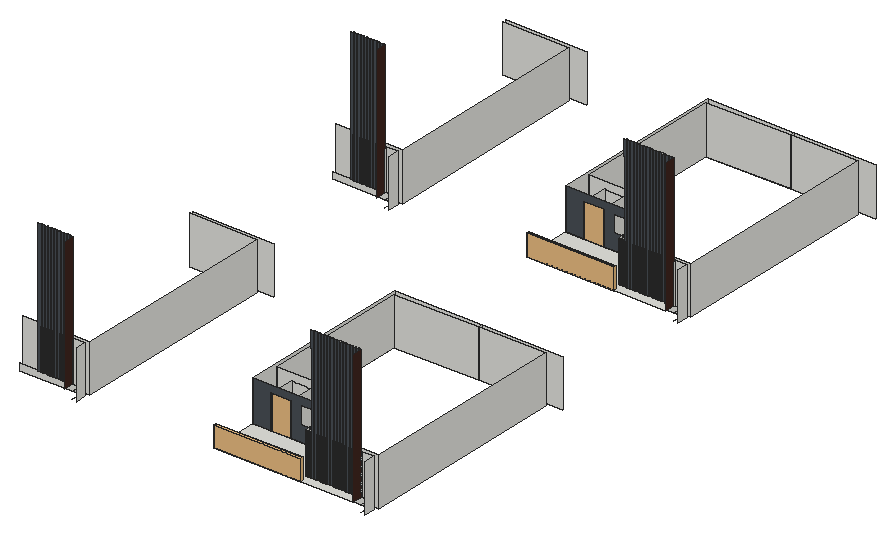
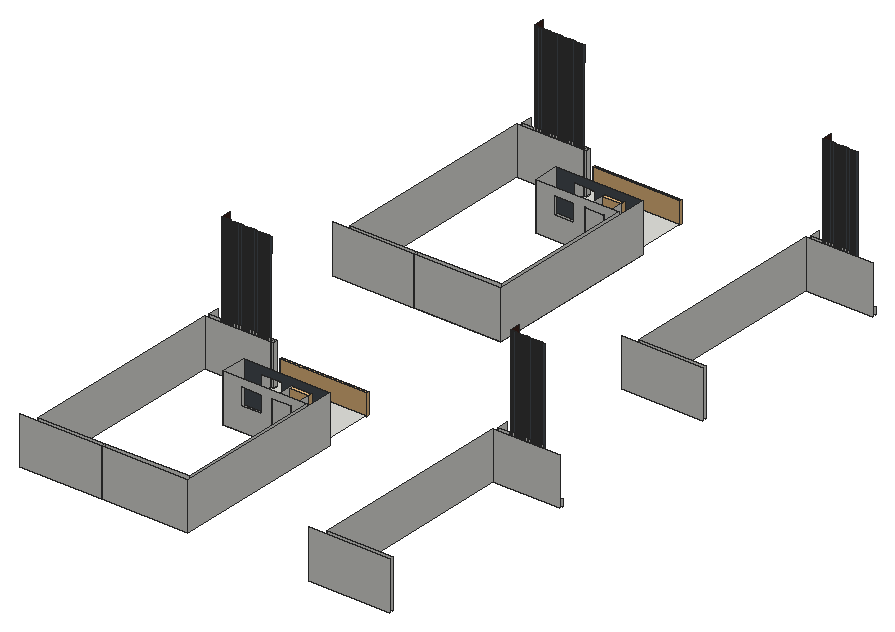
# SketchUp Ruby script. Lengths in inches.
U = 1.inch
M = Sketchup.active_model
def pt(a) = Geom::Point3d.new(a.map { |v| v * U })
def face(e, loops, mat)
  f = e.add_face(loops[0].map { |a| pt(a) })
  loops[1..].each { |l| e.add_face(l.map { |a| pt(a) }).erase! }
  f.material = f.back_material = mat if mat
  f
end
# faces: each face lists its corners as indices into pts; further lists are holes
def faces(e, pts, list, mat = nil) = list.each { |f| face(e, (f[0].is_a?(Array) ? f : [f]).map { |l| l.map { |i| pts[i] } }, mat) }
# xy, xz, yz: faces in a plane at the given z, y or x. An outline is a flat list of corners, or four numbers for a rectangle; further outlines are holes
def ring(l) = l.size == 4 ? [[l[0], l[1]], [l[2], l[1]], [l[2], l[3]], [l[0], l[3]]] : l.each_slice(2).to_a
def flat(e, list, mat, &to3) = list.each { |f| face(e, (f[0].is_a?(Array) ? f : [f]).map { |l| ring(l).map { |u, v| to3.(u, v) } }, mat) }
def xy(e, z, list, mat = nil) = flat(e, list, mat) { |x, y| [x, y, z] }
def xz(e, y, list, mat = nil) = flat(e, list, mat) { |x, z| [x, y, z] }
def yz(e, x, list, mat = nil) = flat(e, list, mat) { |y, z| [x, y, z] }
def lines(e, pts, list) = list.each { |a, b| e.add_line(pt(pts[a]), pt(pts[b])) }
# prism: a flat outline (further loops are holes) pulled along v
def prism(e, loops, v, mat = nil)
  f = face(e, loops, mat); d = Geom::Vector3d.new(v.map { |x| x * U })
  f.pushpull(f.normal.samedirection?(d) ? d.length : -d.length)
end
def box(e, o, s, mat = nil) = prism(e, [[o, [o[0] + s[0], o[1], o[2]], [o[0] + s[0], o[1] + s[1], o[2]], [o[0], o[1] + s[1], o[2]]]], [0, 0, s[2]], mat)
def at(x, y, z, deg = 0) = Geom::Transformation.translation(pt([x, y, z])) * Geom::Transformation.rotation(ORIGIN, Z_AXIS, deg.degrees)
def axes(o, x, y, z) = Geom::Transformation.new([*x, 0, *y, 0, *z, 0, *pt(o).to_a, 1])
def part(name) = M.definitions.add(name)
# library, detail: a bought-in or finely detailed component or shape, given as its bounding box
def library(name, o, s) = part(name).tap { |d| box(d.entities, o, s) }
def detail(e, o, s) = box(e.add_group.entities, o, s)
def put(e, d, t, mat = nil) = e.add_instance(d, t).tap { |i| i.material = mat if mat }
def group(e, t, mat = nil) = e.add_group.tap { |g| g.transformation = t; g.material = mat if mat }.entities
root = M.entities
M.materials.add("[0043_SaddleBrown]").color = [63, 38, 31]
M.materials.add("[Formica Blue]").color = [73, 80, 86]
c1 = library("door (1)",[38.93,25.48,0],[40,9.94,82.68])
c2 = library("Glass Railing",[0,0,0],[139.5,4.76,42])
xy(root,384.25,[[1797.0625,438.72,1802.84,447.84],[1586.375,535.375,1586.375,980.35,1802.84,980.35,1802.84,971.23,1593.72,965.96,1593.72,540.48,1802.84,540.48,1802.84,535.375],[1593.72,540.48,1802.84,598.8125],[1797.0625,1419.07,1802.84,1428.19],[1586.375,1515.73,1586.375,1960.7,1802.84,1960.7,1802.84,1951.58,1593.72,1946.3125,1593.72,1520.83,1802.84,1520.83,1802.84,1515.73],
  [1593.72,1520.83,1802.84,1579.16]])
xy(root,401.6875,[[1586.375,412.04,1935.9375,412.04,1935.9375,437.1,1930.18,437.1,1930.18,438.72,1927.9375,438.72,1927.9375,437.1,1922.18,437.1,1922.18,438.72,1919.9375,438.72,1919.9375,437.1,1914.18,437.1,1914.18,438.72,1911.9375,438.72,1911.9375,437.1,1906.18,437.1,1906.18,438.72,1903.9375,438.72,1903.9375,437.1,1898.18,437.1,1898.18,438.72,1895.9375,438.72,1895.9375,437.1,1890.18,437.1,1890.18,438.72,1887.9375,438.72,1887.9375,437.1,1882.18,437.1,1882.18,438.72,1879.9375,438.72,1879.9375,437.1,1874.18,437.1,1874.18,438.72,1871.9375,438.72,1871.9375,437.1,1866.18,437.1,1866.18,438.72,1863.9375,438.72,1863.9375,437.1,1858.18,437.1,1858.18,438.72,1855.9375,438.72,1855.9375,437.1,1850.18,437.1,1850.18,438.72,1847.9375,438.72,1847.9375,437.1,1842.18,437.1,1842.18,438.72,1839.9375,438.72,1839.9375,437.1,1834.18,437.1,1834.18,438.72,1831.9375,438.72,1831.9375,437.1,1826.18,437.1,1826.18,438.72,1823.9375,438.72,1823.9375,437.1,1818.18,437.1,1818.18,438.72,1815.9375,438.72,1815.9375,437.1,1810.18,437.1,1810.18,438.72,1807.75,438.72,1807.75,437.1,1802.84,437.1,1802.84,438.72,1801.29,438.72,1801.29,437.1,1797.0625,437.1,1797.0625,447.84,1802.84,447.84,1802.84,535.375,1586.375,535.375],[1133.74,437.1,1139.5,438.72],[1141.74,437.1,1147.5,438.72],[1149.74,437.1,1155.5,438.72],[1157.74,437.1,1163.5,438.72],
  [1165.74,437.1,1171.5,438.72],[1173.74,437.1,1179.5,438.72],[1181.74,437.1,1187.5,438.72],[1189.74,437.1,1195.5,438.72],[1197.74,437.1,1203.5,438.72],
  [1205.74,437.1,1211.5,438.72],[1797.0625,437.1,1801.29,438.72],[1802.84,437.1,1807.75,438.72],[1810.18,437.1,1815.9375,438.72],[1818.18,437.1,1823.9375,438.72],
  [1826.18,437.1,1831.9375,438.72],[1834.18,437.1,1839.9375,438.72],[1842.18,437.1,1847.9375,438.72],[1850.18,437.1,1855.9375,438.72],[1858.18,437.1,1863.9375,438.72],
  [1866.18,437.1,1871.9375,438.72],[1874.18,437.1,1879.9375,438.72],[1882.18,437.1,1887.9375,438.72],[1890.18,437.1,1895.9375,438.72],[1898.18,437.1,1903.9375,438.72],
  [1906.18,437.1,1911.9375,438.72],[1914.18,437.1,1919.9375,438.72],[1922.18,437.1,1927.9375,438.72],[1930.18,437.1,1935.9375,438.72],[1632.17,535.375,1680.17,598.8125],
  [1586.375,1392.39,1935.9375,1392.39,1935.9375,1417.45,1930.18,1417.45,1930.18,1419.07,1927.9375,1419.07,1927.9375,1417.45,1922.18,1417.45,1922.18,1419.07,1919.9375,1419.07,1919.9375,1417.45,1914.18,1417.45,1914.18,1419.07,1911.9375,1419.07,1911.9375,1417.45,1906.18,1417.45,1906.18,1419.07,1903.9375,1419.07,1903.9375,1417.45,1898.18,1417.45,1898.18,1419.07,1895.9375,1419.07,1895.9375,1417.45,1890.18,1417.45,1890.18,1419.07,1887.9375,1419.07,1887.9375,1417.45,1882.18,1417.45,1882.18,1419.07,1879.9375,1419.07,1879.9375,1417.45,1874.18,1417.45,1874.18,1419.07,1871.9375,1419.07,1871.9375,1417.45,1866.18,1417.45,1866.18,1419.07,1863.9375,1419.07,1863.9375,1417.45,1858.18,1417.45,1858.18,1419.07,1855.9375,1419.07,1855.9375,1417.45,1850.18,1417.45,1850.18,1419.07,1847.9375,1419.07,1847.9375,1417.45,1842.18,1417.45,1842.18,1419.07,1839.9375,1419.07,1839.9375,1417.45,1834.18,1417.45,1834.18,1419.07,1831.9375,1419.07,1831.9375,1417.45,1826.18,1417.45,1826.18,1419.07,1823.9375,1419.07,1823.9375,1417.45,1818.18,1417.45,1818.18,1419.07,1815.9375,1419.07,1815.9375,1417.45,1810.18,1417.45,1810.18,1419.07,1807.75,1419.07,1807.75,1417.45,1802.84,1417.45,1802.84,1419.07,1801.29,1419.07,1801.29,1417.45,1797.0625,1417.45,1797.0625,1428.19,1802.84,1428.19,1802.84,1515.73,1586.375,1515.73],[1125.74,1417.45,1131.5,1419.07],[1133.74,1417.45,1139.5,1419.07],[1141.74,1417.45,1147.5,1419.07],[1149.74,1417.45,1155.5,1419.07],
  [1157.74,1417.45,1163.5,1419.07],[1165.74,1417.45,1171.5,1419.07],[1173.74,1417.45,1179.5,1419.07],[1181.74,1417.45,1187.5,1419.07],[1189.74,1417.45,1195.5,1419.07],
  [1197.74,1417.45,1203.5,1419.07],[1205.74,1417.45,1211.5,1419.07],[1797.0625,1417.45,1801.29,1419.07],[1802.84,1417.45,1807.75,1419.07],[1810.18,1417.45,1815.9375,1419.07],
  [1818.18,1417.45,1823.9375,1419.07],[1826.18,1417.45,1831.9375,1419.07],[1834.18,1417.45,1839.9375,1419.07],[1842.18,1417.45,1847.9375,1419.07],[1850.18,1417.45,1855.9375,1419.07],
  [1858.18,1417.45,1863.9375,1419.07],[1866.18,1417.45,1871.9375,1419.07],[1874.18,1417.45,1879.9375,1419.07],[1882.18,1417.45,1887.9375,1419.07],[1890.18,1417.45,1895.9375,1419.07],
  [1898.18,1417.45,1903.9375,1419.07],[1906.18,1417.45,1911.9375,1419.07],[1914.18,1417.45,1919.9375,1419.07],[1922.18,1417.45,1927.9375,1419.07],[1930.18,1417.45,1935.9375,1419.07],
  [1632.17,1515.73,1680.17,1579.16]])
xz(root,437.1,[[1125.74,401.6875,1131.5,733.125],[1133.74,401.6875,1139.5,733.125],[1141.74,401.6875,1147.5,733.125],[1149.74,401.6875,1155.5,733.125],[1157.74,401.6875,1163.5,733.125],
  [1165.74,401.6875,1171.5,733.125],[1173.74,401.6875,1179.5,733.125],[1181.74,401.6875,1187.5,733.125],[1189.74,401.6875,1195.5,733.125],[1197.74,401.6875,1203.5,733.125],
  [1205.74,401.6875,1211.5,733.125],[1797.0625,401.6875,1801.29,504.25],[1802.84,401.6875,1807.75,504.25],[1810.18,401.6875,1815.9375,401.6875,1815.9375,733.125,1810.18,733.125,1810.18,693.65,1812.6,693.65,1812.6,504.25,1810.18,504.25],[1818.18,401.6875,1823.9375,733.125],
  [1826.18,401.6875,1831.9375,733.125],[1834.18,401.6875,1839.9375,733.125],[1842.18,401.6875,1847.9375,733.125],[1850.18,401.6875,1855.9375,733.125],[1858.18,401.6875,1863.9375,733.125],
  [1866.18,401.6875,1871.9375,733.125],[1874.18,401.6875,1879.9375,733.125],[1882.18,401.6875,1887.9375,733.125],[1890.18,401.6875,1895.9375,733.125],[1898.18,401.6875,1903.9375,733.125],
  [1906.18,401.6875,1911.9375,733.125],[1914.18,401.6875,1919.9375,733.125],[1922.18,401.6875,1927.9375,733.125],[1930.18,401.6875,1935.9375,733.125]],"[Formica Blue]")
xz(root,438.72,[[1078.41,384.25,1228.9375,401.6875],[1797.0625,384.25,1802.84,401.6875],[1802.84,384.25,1953.375,401.6875]])
xz(root,438.72,[[1131.5,401.6875,1133.74,733.125],[1139.5,401.6875,1141.74,733.125],[1147.5,401.6875,1149.74,733.125],[1155.5,401.6875,1157.74,733.125],[1163.5,401.6875,1165.74,733.125],
  [1171.5,401.6875,1173.74,733.125],[1179.5,401.6875,1181.74,733.125],[1187.5,401.6875,1189.74,733.125],[1195.5,401.6875,1197.74,733.125],[1203.5,401.6875,1205.74,733.125],
  [1801.29,401.6875,1802.84,504.25],[1807.75,401.6875,1810.18,504.25],[1815.9375,401.6875,1818.18,733.125],[1823.9375,401.6875,1826.18,733.125],[1831.9375,401.6875,1834.18,733.125],
  [1839.9375,401.6875,1842.18,733.125],[1847.9375,401.6875,1850.18,733.125],[1855.9375,401.6875,1858.18,733.125],[1863.9375,401.6875,1866.18,733.125],[1871.9375,401.6875,1874.18,733.125],
  [1879.9375,401.6875,1882.18,733.125],[1887.9375,401.6875,1890.18,733.125],[1895.9375,401.6875,1898.18,733.125],[1903.9375,401.6875,1906.18,733.125],[1911.9375,401.6875,1914.18,733.125],
  [1919.9375,401.6875,1922.18,733.125],[1927.9375,401.6875,1930.18,733.125]],"[Formica Blue]")
xz(root,447.84,[[1078.41,384.25,1246.07,504.25],[1797.0625,384.25,1802.84,401.6875],[1802.84,384.25,1970.51,504.25],[1797.0625,401.6875,1802.84,504.25]])
xz(root,535.375,[[1586.375,384.25,1802.84,401.6875]])
xz(root,535.375,[[[1586.375,401.6875,1632.17,401.6875,1632.17,485.6875,1680.17,485.6875,1680.17,401.6875,1802.84,401.6875,1802.84,504.25,1586.375,504.25],[1706.96,441.5,1758.71,485.6875]]],"[Formica Blue]")
xz(root,598.8125,[[[1593.72,384.25,1802.84,504.25],[1632.17,401.6875,1680.17,485.6875],[1706.96,441.5,1758.71,485.6875]],[1632.17,401.6875,1680.17,485.6875]])
xz(root,971.23,[[1078.41,384.25,1246.07,504.25],[1802.84,384.25,1970.51,504.25]])
xz(root,980.35,[[1078.41,384.25,1283.0625,504.25],[1586.375,384.25,1802.84,504.25],[1802.84,384.25,2007.5,504.25]])
xz(root,1417.45,[[1125.74,401.6875,1131.5,733.125],[1133.74,401.6875,1139.5,733.125],[1141.74,401.6875,1147.5,733.125],[1149.74,401.6875,1155.5,733.125],[1157.74,401.6875,1163.5,733.125],
  [1165.74,401.6875,1171.5,733.125],[1173.74,401.6875,1179.5,733.125],[1181.74,401.6875,1187.5,733.125],[1189.74,401.6875,1195.5,733.125],[1197.74,401.6875,1203.5,733.125],
  [1205.74,401.6875,1211.5,733.125],[1797.0625,401.6875,1801.29,504.25],[1802.84,401.6875,1807.75,504.25],[1810.18,401.6875,1815.9375,401.6875,1815.9375,733.125,1810.18,733.125,1810.18,693.65,1812.6,693.65,1812.6,504.25,1810.18,504.25],[1818.18,401.6875,1823.9375,733.125],
  [1826.18,401.6875,1831.9375,733.125],[1834.18,401.6875,1839.9375,733.125],[1842.18,401.6875,1847.9375,733.125],[1850.18,401.6875,1855.9375,733.125],[1858.18,401.6875,1863.9375,733.125],
  [1866.18,401.6875,1871.9375,733.125],[1874.18,401.6875,1879.9375,733.125],[1882.18,401.6875,1887.9375,733.125],[1890.18,401.6875,1895.9375,733.125],[1898.18,401.6875,1903.9375,733.125],
  [1906.18,401.6875,1911.9375,733.125],[1914.18,401.6875,1919.9375,733.125],[1922.18,401.6875,1927.9375,733.125],[1930.18,401.6875,1935.9375,733.125]],"[Formica Blue]")
xz(root,1419.07,[[1078.41,384.25,1228.9375,401.6875],[1797.0625,384.25,1802.84,401.6875],[1802.84,384.25,1953.375,401.6875]])
xz(root,1419.07,[[1131.5,401.6875,1133.74,733.125],[1139.5,401.6875,1141.74,733.125],[1147.5,401.6875,1149.74,733.125],[1155.5,401.6875,1157.74,733.125],[1163.5,401.6875,1165.74,733.125],
  [1171.5,401.6875,1173.74,733.125],[1179.5,401.6875,1181.74,733.125],[1187.5,401.6875,1189.74,733.125],[1195.5,401.6875,1197.74,733.125],[1203.5,401.6875,1205.74,733.125],
  [1801.29,401.6875,1802.84,504.25],[1807.75,401.6875,1810.18,504.25],[1815.9375,401.6875,1818.18,733.125],[1823.9375,401.6875,1826.18,733.125],[1831.9375,401.6875,1834.18,733.125],
  [1839.9375,401.6875,1842.18,733.125],[1847.9375,401.6875,1850.18,733.125],[1855.9375,401.6875,1858.18,733.125],[1863.9375,401.6875,1866.18,733.125],[1871.9375,401.6875,1874.18,733.125],
  [1879.9375,401.6875,1882.18,733.125],[1887.9375,401.6875,1890.18,733.125],[1895.9375,401.6875,1898.18,733.125],[1903.9375,401.6875,1906.18,733.125],[1911.9375,401.6875,1914.18,733.125],
  [1919.9375,401.6875,1922.18,733.125],[1927.9375,401.6875,1930.18,733.125]],"[Formica Blue]")
xz(root,1428.19,[[1078.41,384.25,1246.07,504.25],[1797.0625,384.25,1802.84,401.6875],[1802.84,384.25,1970.51,504.25],[1797.0625,401.6875,1802.84,504.25]])
xz(root,1515.73,[[1586.375,384.25,1802.84,401.6875]])
xz(root,1515.73,[[[1586.375,401.6875,1632.17,401.6875,1632.17,485.6875,1680.17,485.6875,1680.17,401.6875,1802.84,401.6875,1802.84,504.25,1586.375,504.25],[1706.96,441.5,1758.71,485.6875]]],"[Formica Blue]")
xz(root,1579.16,[[[1593.72,384.25,1802.84,504.25],[1632.17,401.6875,1680.17,485.6875],[1706.96,441.5,1758.71,485.6875]],[1632.17,401.6875,1680.17,485.6875]])
xz(root,1951.58,[[1078.41,384.25,1246.07,504.25],[1802.84,384.25,1970.51,504.25]])
xz(root,1960.7,[[1078.41,384.25,1283.0625,504.25],[1586.375,384.25,1802.84,504.25],[1802.84,384.25,2007.5,504.25]])
yz(root,1131.5,[[437.1,401.6875,438.72,504.25],[1417.45,401.6875,1419.07,504.25]])
yz(root,1133.74,[[437.1,401.6875,438.72,733.125],[1417.45,401.6875,1419.07,733.125]])
yz(root,1139.5,[[437.1,401.6875,438.72,504.25],[1417.45,401.6875,1419.07,504.25]])
yz(root,1141.74,[[437.1,401.6875,438.72,733.125],[1417.45,401.6875,1419.07,733.125]])
yz(root,1147.5,[[437.1,401.6875,438.72,504.25],[1417.45,401.6875,1419.07,504.25]])
yz(root,1149.74,[[437.1,401.6875,438.72,733.125],[1417.45,401.6875,1419.07,733.125]])
yz(root,1155.5,[[437.1,401.6875,438.72,504.25],[1417.45,401.6875,1419.07,504.25]])
yz(root,1157.74,[[437.1,401.6875,438.72,733.125],[1417.45,401.6875,1419.07,733.125]])
yz(root,1163.5,[[437.1,401.6875,438.72,504.25],[1417.45,401.6875,1419.07,504.25]])
yz(root,1165.74,[[437.1,401.6875,438.72,733.125],[1417.45,401.6875,1419.07,733.125]])
yz(root,1171.5,[[437.1,401.6875,438.72,504.25],[1417.45,401.6875,1419.07,504.25]])
yz(root,1173.74,[[437.1,401.6875,438.72,733.125],[1417.45,401.6875,1419.07,733.125]])
yz(root,1179.5,[[437.1,401.6875,438.72,504.25],[1417.45,401.6875,1419.07,504.25]])
yz(root,1181.74,[[437.1,401.6875,438.72,733.125],[1417.45,401.6875,1419.07,733.125]])
yz(root,1187.5,[[437.1,401.6875,438.72,504.25],[1417.45,401.6875,1419.07,504.25]])
yz(root,1189.74,[[437.1,401.6875,438.72,733.125],[1417.45,401.6875,1419.07,733.125]])
yz(root,1195.5,[[437.1,401.6875,438.72,504.25],[1417.45,401.6875,1419.07,504.25]])
yz(root,1197.74,[[437.1,401.6875,438.72,733.125],[1417.45,401.6875,1419.07,733.125]])
yz(root,1203.5,[[437.1,401.6875,438.72,504.25],[1417.45,401.6875,1419.07,504.25]])
yz(root,1205.74,[[437.1,401.6875,438.72,733.125],[1417.45,401.6875,1419.07,733.125]])
yz(root,1211.5,[[437.1,401.6875,438.72,504.25],[1417.45,401.6875,1419.07,504.25]])
yz(root,1211.5,[[412.04,401.6875,437.1,733.125],[1392.39,401.6875,1417.45,733.125]],"[0043_SaddleBrown]")
yz(root,1241.75,[[412.04,384.25,438.72,384.25,438.73,409.48,438.72,412.48,438.72,504.25,412.04,504.25],[1392.39,384.25,1419.07,384.25,1419.08,409.48,1419.07,412.48,1419.07,504.25,1392.39,504.25]])
yz(root,1246.07,[[447.84,384.25,971.23,504.25],[1428.19,384.25,1951.58,504.25]])
yz(root,1586.375,[[535.375,384.25,980.35,504.25],[1515.73,384.25,1960.7,504.25]])
yz(root,1593.72,[[598.8125,384.25,965.96,504.25],[1579.16,384.25,1946.3125,504.25]])
yz(root,1632.17,[[535.375,401.6875,598.8125,485.6875],[1515.73,401.6875,1579.16,485.6875]])
yz(root,1680.17,[[535.375,401.6875,598.8125,485.6875],[1515.73,401.6875,1579.16,485.6875]])
yz(root,1797.0625,[[438.72,384.25,447.84,401.6875],[1419.07,384.25,1428.19,401.6875],[437.1,401.6875,447.84,504.25],[1417.45,401.6875,1428.19,504.25]])
yz(root,1801.29,[[437.1,401.6875,438.72,504.25],[1417.45,401.6875,1419.07,504.25]])
yz(root,1802.84,[[438.72,384.25,447.84,504.25],[535.375,384.25,598.8125,504.25],[971.23,384.25,980.35,504.25],[1419.07,384.25,1428.19,504.25],[1515.73,384.25,1579.16,504.25],
  [1951.58,384.25,1960.7,504.25],[437.1,401.6875,438.72,504.25],[1417.45,401.6875,1419.07,504.25]])
yz(root,1807.75,[[437.1,401.6875,438.72,504.25],[1417.45,401.6875,1419.07,504.25]])
yz(root,1810.18,[[437.1,401.6875,438.72,504.25],[1417.45,401.6875,1419.07,504.25]])
yz(root,1815.9375,[[437.1,401.6875,438.72,504.25],[1417.45,401.6875,1419.07,504.25]])
yz(root,1818.18,[[437.1,401.6875,438.72,733.125],[1417.45,401.6875,1419.07,733.125]])
yz(root,1823.9375,[[437.1,401.6875,438.72,504.25],[1417.45,401.6875,1419.07,504.25]])
yz(root,1826.18,[[437.1,401.6875,438.72,733.125],[1417.45,401.6875,1419.07,733.125]])
yz(root,1831.9375,[[437.1,401.6875,438.72,504.25],[1417.45,401.6875,1419.07,504.25]])
yz(root,1834.18,[[437.1,401.6875,438.72,733.125],[1417.45,401.6875,1419.07,733.125]])
yz(root,1839.9375,[[437.1,401.6875,438.72,504.25],[1417.45,401.6875,1419.07,504.25]])
yz(root,1842.18,[[437.1,401.6875,438.72,733.125],[1417.45,401.6875,1419.07,733.125]])
yz(root,1847.9375,[[437.1,401.6875,438.72,504.25],[1417.45,401.6875,1419.07,504.25]])
yz(root,1850.18,[[437.1,401.6875,438.72,733.125],[1417.45,401.6875,1419.07,733.125]])
yz(root,1855.9375,[[437.1,401.6875,438.72,504.25],[1417.45,401.6875,1419.07,504.25]])
yz(root,1858.18,[[437.1,401.6875,438.72,733.125],[1417.45,401.6875,1419.07,733.125]])
yz(root,1863.9375,[[437.1,401.6875,438.72,504.25],[1417.45,401.6875,1419.07,504.25]])
yz(root,1866.18,[[437.1,401.6875,438.72,733.125],[1417.45,401.6875,1419.07,733.125]])
yz(root,1871.9375,[[437.1,401.6875,438.72,504.25],[1417.45,401.6875,1419.07,504.25]])
yz(root,1874.18,[[437.1,401.6875,438.72,733.125],[1417.45,401.6875,1419.07,733.125]])
yz(root,1879.9375,[[437.1,401.6875,438.72,504.25],[1417.45,401.6875,1419.07,504.25]])
yz(root,1882.18,[[437.1,401.6875,438.72,733.125],[1417.45,401.6875,1419.07,733.125]])
yz(root,1887.9375,[[437.1,401.6875,438.72,504.25],[1417.45,401.6875,1419.07,504.25]])
yz(root,1890.18,[[437.1,401.6875,438.72,733.125],[1417.45,401.6875,1419.07,733.125]])
yz(root,1895.9375,[[437.1,401.6875,438.72,504.25],[1417.45,401.6875,1419.07,504.25]])
yz(root,1898.18,[[437.1,401.6875,438.72,733.125],[1417.45,401.6875,1419.07,733.125]])
yz(root,1903.9375,[[437.1,401.6875,438.72,504.25],[1417.45,401.6875,1419.07,504.25]])
yz(root,1906.18,[[437.1,401.6875,438.72,733.125],[1417.45,401.6875,1419.07,733.125]])
yz(root,1911.9375,[[437.1,401.6875,438.72,504.25],[1417.45,401.6875,1419.07,504.25]])
yz(root,1914.18,[[437.1,401.6875,438.72,733.125],[1417.45,401.6875,1419.07,733.125]])
yz(root,1919.9375,[[437.1,401.6875,438.72,504.25],[1417.45,401.6875,1419.07,504.25]])
yz(root,1922.18,[[437.1,401.6875,438.72,733.125],[1417.45,401.6875,1419.07,733.125]])
yz(root,1927.9375,[[437.1,401.6875,438.72,504.25],[1417.45,401.6875,1419.07,504.25]])
yz(root,1930.18,[[437.1,401.6875,438.72,733.125],[1417.45,401.6875,1419.07,733.125]])
yz(root,1935.9375,[[437.1,401.6875,438.72,504.25],[1417.45,401.6875,1419.07,504.25]])
yz(root,1935.9375,[[412.04,401.6875,437.1,733.125],[1392.39,401.6875,1417.45,733.125]],"[0043_SaddleBrown]")
yz(root,1966.1875,[[412.04,384.25,438.72,384.25,438.73,409.48,438.72,412.48,438.72,504.25,412.04,504.25],[1392.39,384.25,1419.07,384.25,1419.08,409.48,1419.07,412.48,1419.07,504.25,1392.39,504.25]])
yz(root,1970.51,[[447.84,384.25,971.23,504.25],[1428.19,384.25,1951.58,504.25]])
p = [[1228.9375,438.72,384.25],[1241.75,438.72,384.25],[1241.75,438.73,409.48],[1241.75,438.72,412.48],[1241.75,438.72,504.25],[1211.5,438.72,504.25],
  [1211.5,438.72,401.6875],[1228.9375,438.72,401.6875],[1953.375,438.72,384.25],[1966.1875,438.72,384.25],[1966.1875,438.73,409.48],[1966.1875,438.72,412.48],
  [1966.1875,438.72,504.25],[1935.9375,438.72,504.25],[1935.9375,438.72,401.6875],[1953.375,438.72,401.6875],[1593.72,965.96,384.25],[1802.84,971.23,384.25],
  [1802.84,971.23,504.25],[1593.72,965.96,504.25],[1228.9375,1419.07,384.25],[1241.75,1419.07,384.25],[1241.75,1419.08,409.48],[1241.75,1419.07,412.48],
  [1241.75,1419.07,504.25],[1211.5,1419.07,504.25],[1211.5,1419.07,401.6875],[1228.9375,1419.07,401.6875],[1953.375,1419.07,384.25],[1966.1875,1419.07,384.25],
  [1966.1875,1419.08,409.48],[1966.1875,1419.07,412.48],[1966.1875,1419.07,504.25],[1935.9375,1419.07,504.25],[1935.9375,1419.07,401.6875],[1953.375,1419.07,401.6875],
  [1593.72,1946.3125,384.25],[1802.84,1951.58,384.25],[1802.84,1951.58,504.25],[1593.72,1946.3125,504.25],[1228.9375,412.04,384.25],[1228.9375,412.04,401.6875],
  [1953.375,412.04,401.6875],[1953.375,412.04,384.25],[1228.9375,1392.39,384.25],[1228.9375,1392.39,401.6875],[1953.375,1392.39,401.6875],[1953.375,1392.39,384.25]]
faces(root,p,[[0,1,2,3,4,5,6,7],[8,9,10,11,12,13,14,15],[16,17,18,19],[20,21,22,23,24,25,26,27],[28,29,30,31,32,33,34,35],[36,37,38,39]])
lines(root,p,[[0,40],[7,41],[15,42],[8,43],[20,44],[27,45],[35,46],[28,47]])
put(root,c1,axes([1582.69,1490.24,401.6875],[1.2351,0,0],[0,1,0],[0,0,1.016]))
put(root,c1,axes([1582.69,509.89,401.6875],[1.2351,0,0],[0,1,0],[0,0,1.016]))
put(root,c2,axes([1586.375,413.41,399.63],[1.55466,0,0],[0,1.27,0],[0,0,1.27]))
put(root,c2,axes([1586.375,1393.76,399.63],[1.55466,0,0],[0,1.27,0],[0,0,1.27]))
